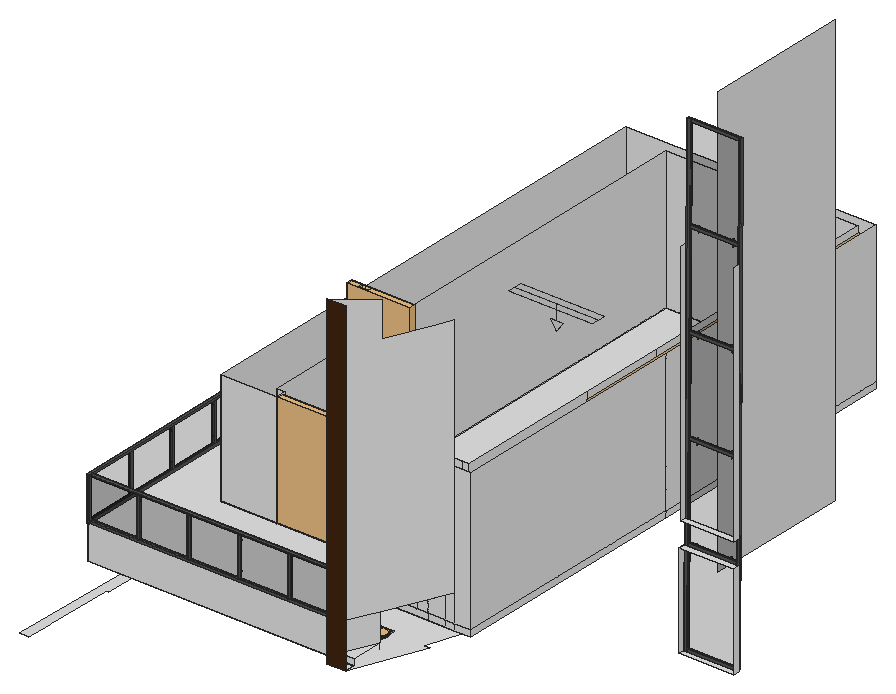
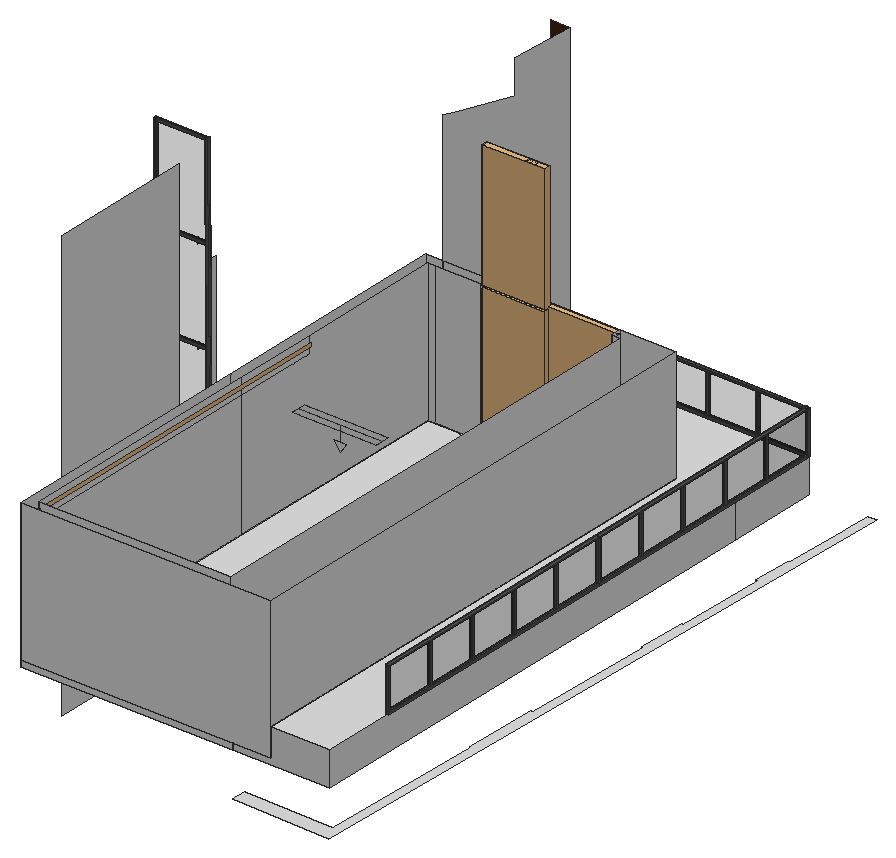
# SketchUp Ruby script. Lengths in inches.
U = 1.inch
M = Sketchup.active_model
def pt(a) = Geom::Point3d.new(a.map { |v| v * U })
def face(e, loops, mat)
  f = e.add_face(loops[0].map { |a| pt(a) })
  loops[1..].each { |l| e.add_face(l.map { |a| pt(a) }).erase! }
  f.material = f.back_material = mat if mat
  f
end
# faces: each face lists its corners as indices into pts; further lists are holes
def faces(e, pts, list, mat = nil) = list.each { |f| face(e, (f[0].is_a?(Array) ? f : [f]).map { |l| l.map { |i| pts[i] } }, mat) }
# xy, xz, yz: faces in a plane at the given z, y or x. An outline is a flat list of corners, or four numbers for a rectangle; further outlines are holes
def ring(l) = l.size == 4 ? [[l[0], l[1]], [l[2], l[1]], [l[2], l[3]], [l[0], l[3]]] : l.each_slice(2).to_a
def flat(e, list, mat, &to3) = list.each { |f| face(e, (f[0].is_a?(Array) ? f : [f]).map { |l| ring(l).map { |u, v| to3.(u, v) } }, mat) }
def xy(e, z, list, mat = nil) = flat(e, list, mat) { |x, y| [x, y, z] }
def xz(e, y, list, mat = nil) = flat(e, list, mat) { |x, z| [x, y, z] }
def yz(e, x, list, mat = nil) = flat(e, list, mat) { |y, z| [x, y, z] }
def lines(e, pts, list) = list.each { |a, b| e.add_line(pt(pts[a]), pt(pts[b])) }
# prism: a flat outline (further loops are holes) pulled along v
def prism(e, loops, v, mat = nil)
  f = face(e, loops, mat); d = Geom::Vector3d.new(v.map { |x| x * U })
  f.pushpull(f.normal.samedirection?(d) ? d.length : -d.length)
end
def box(e, o, s, mat = nil) = prism(e, [[o, [o[0] + s[0], o[1], o[2]], [o[0] + s[0], o[1] + s[1], o[2]], [o[0], o[1] + s[1], o[2]]]], [0, 0, s[2]], mat)
def at(x, y, z, deg = 0) = Geom::Transformation.translation(pt([x, y, z])) * Geom::Transformation.rotation(ORIGIN, Z_AXIS, deg.degrees)
def axes(o, x, y, z) = Geom::Transformation.new([*x, 0, *y, 0, *z, 0, *pt(o).to_a, 1])
def part(name) = M.definitions.add(name)
# library, detail: a bought-in or finely detailed component or shape, given as its bounding box
def library(name, o, s) = part(name).tap { |d| box(d.entities, o, s) }
def detail(e, o, s) = box(e.add_group.entities, o, s)
def put(e, d, t, mat = nil) = e.add_instance(d, t).tap { |i| i.material = mat if mat }
def group(e, t, mat = nil) = e.add_group.tap { |g| g.transformation = t; g.material = mat if mat }.entities
root = M.entities
M.materials.add("Aluminum_Polished").color = [83, 85, 85]
M.materials.add("Glass_Window_Neutral").color = [0, 0, 0]
M.materials["Glass_Window_Neutral"].alpha = 0.125
M.materials.add("Material~1").color = [0, 0, 0]
M.materials.add("[Color M03]").color = [226, 226, 226]
M.materials.add("[Color_001]").color = [196, 196, 196]
M.materials["[Color_001]"].alpha = 0.97
M.materials.add("[Wood Cherry Original]1").color = [66, 37, 18]
c1 = part("Group\#54")
box(c1.entities,[0,0,0],[2,1,28])
c2 = part("Group\#56")
p = [[0.11,0.32,0.14],[0.11,0.69,0.14]]
lines(c2.entities,p,[[0,1]])
g1 = group(c2.entities,at(0.11,0,0))
prism(g1,[[[0,0.24,0],[0,0.32,0.14],[0,0.24,0.27],[0,0.08,0.27],[0,0,0.14],[0,0.08,0]]],[-0.11,0,0])
c3 = part("Ver Glass Railing")
g2 = group(c3.entities,at(0,0,0),"Aluminum_Polished")
box(g2,[0,0,0],[2,185,2])
g3 = group(c3.entities,at(0,0,2),"Aluminum_Polished")
p = [[1.41,1,0],[1.41,36.8,0],[1.41,184,0],[1.29,184,0],[1.29,1,0],[1.29,36.8,0],
  [1.41,184,28],[1.29,184,28],[1.41,148.2,28],[1.29,148.2,28],[1.41,1,28],[1.29,1,28],
  [1.29,111.4,28],[1.29,111.4,0],[1.41,111.4,0],[1.41,111.4,28],[1.29,110.4,0],[1.29,110.4,28],
  [1.41,110.4,28],[1.41,110.4,0],[1.29,74.6,28],[1.29,74.6,0],[1.41,74.6,0],[1.41,74.6,28],
  [1.29,73.6,0],[1.29,73.6,28],[1.41,73.6,28],[1.41,73.6,0],[1.29,148.2,0],[1.41,148.2,0],
  [1.29,147.2,0],[1.29,147.2,28],[1.41,147.2,28],[1.41,147.2,0],[1.29,37.8,28],[1.29,37.8,0],
  [1.41,37.8,0],[1.41,37.8,28],[1.29,36.8,28],[1.41,36.8,28]]
lines(g3,p,[[0,1],[2,3],[4,5],[6,7],[6,8],[7,9],[10,11],[2,6],[3,7],[0,4],[11,4],[10,0],
  [12,13],[14,15],[16,17],[18,19],[20,21],[22,23],[24,25],[26,27],[27,22],[24,21],[23,26],[20,25],
  [9,28],[29,8],[30,31],[32,33],[33,29],[30,28],[8,32],[9,31],[34,35],[36,37],[5,38],[39,1],
  [1,36],[5,35],[37,39],[14,33],[19,14],[22,19],[36,27],[13,30],[16,13],[21,16],[35,24],[15,18],
  [12,17],[29,2],[28,3],[18,23],[32,15],[17,20],[31,12],[26,37],[25,34],[34,38],[39,10],[38,11]])
g4 = group(g3,at(1.79,1,0))
box(g4,[-0.5,0,0],[0.125,183,28],"Glass_Window_Neutral")
g5 = group(g3,at(0,184,28))
box(g5,[0,-184,0],[2.5,185,1])
put(g3,c1,axes([2,185,28],[-1,0,0],[0,-1,0],[0,0,-1]))
put(g3,c1,axes([2,1,28],[-1,0,0],[0,-1,0],[0,0,-1]))
put(g3,c1,axes([2,111.4,28],[-1,0,0],[0,-1,0],[0,0,-1]))
put(g3,c1,axes([2,74.6,28],[-1,0,0],[0,-1,0],[0,0,-1]))
g6 = group(g3,at(2,148.2,28))
box(g6,[-2,-1,-28],[2,1,28])
put(g3,c1,axes([2,37.8,28],[-1,0,0],[0,-1,0],[0,0,-1]))
put(g3,c2,at(1.17,146.31,24.26))
put(g3,c2,axes([1.17,148.89,24.54],[1,0,0],[0,-1,0],[0,0,-1]))
put(g3,c2,axes([1.17,148.89,4.79],[1,0,0],[0,-1,0],[0,0,-1]))
put(g3,c2,at(1.17,146.31,4.51))
put(g3,c2,at(1.17,109.51,4.51))
put(g3,c2,axes([1.17,112.09,4.79],[1,0,0],[0,-1,0],[0,0,-1]))
put(g3,c2,axes([1.17,112.09,24.54],[1,0,0],[0,-1,0],[0,0,-1]))
put(g3,c2,at(1.17,109.51,24.26))
put(g3,c2,axes([1.17,75.29,24.54],[1,0,0],[0,-1,0],[0,0,-1]))
put(g3,c2,at(1.17,72.71,4.51))
put(g3,c2,axes([1.17,75.29,4.79],[1,0,0],[0,-1,0],[0,0,-1]))
put(g3,c2,at(1.17,72.71,24.26))
put(g3,c2,axes([1.17,38.49,24.54],[1,0,0],[0,-1,0],[0,0,-1]))
put(g3,c2,at(1.17,35.91,4.51))
put(g3,c2,axes([1.17,38.49,4.79],[1,0,0],[0,-1,0],[0,0,-1]))
put(g3,c2,at(1.17,35.91,24.26))
c4 = part("Group259\#1")
p = [[0,0,0],[0,0,-6.22],[-2.62,0,-6.22],[17.05,-3.08,0],[-17.05,-3.08,0],[17.05,3.08,0],
  [17.05,0,0],[-17.05,3.08,0],[2.62,0,-6.22],[-17.05,0,0],[0,0,-10.0625]]
lines(c4.entities,p,[[0,1],[1,2],[3,4],[5,6],[7,5],[1,8],[9,0],[0,6],[8,10],[4,9],[6,3],[2,10],
  [9,7]])
c5 = part("Rectangle Light\#1")
put(c5.entities,c4,at(0,0,0))
c6 = library("Spot Light",[-5.1,-5.1,-11.05],[10.2,10.2,11.05])
c7 = library("Mesh Light\#8",[-0.5,-0.5,-0.1],[1,1,0.2])
c8 = library("Group\#3",[-0.5,-0.5,-0.1],[13,13,0.2])
c9 = library("Group11\#3",[-63.24,494.46,2.3125],[92.6,100.74,2109.15])
c10 = library("3DGeom~3_Defintion\#7",[-166.03,-457.45,-50.66],[409.15,1000,95.96])
c11 = part("Group12\#3")
put(c11.entities,c10,axes([-25.11,656.6,967.09],[0,1.68483,0],[0,0,2.10997],[-1.81292,0,0]),"Material~1")
c12 = part("Group10\#3")
put(c12.entities,c9,at(0,0,0),"[Color_001]")
put(c12.entities,c11,at(0,0,0))
c13 = library("Sliding Door",[0,0,0],[94.49,5.83,91.73])
c14 = library("Mesh Light\#7",[-0.5,-0.5,-0.1],[1,1,0.2])
xy(root,53.02,[[563.22,466.93,616.16,472.23]],"[Color M03]")
xy(root,123.23,[[244.05,83.53,244.68,107.8,243.62,107.83,245.35,174.72,247.41,174.67,248.39,212.13,246.32,212.18,248.6,299.78,250.22,299.74,251.43,346.17,249.8,346.21,253.15,475.08,254.77,475.04,256.62,546.02,254.99,546.0625,259.2,708.3,345.63,706.05,346,720.04,251.84,722.48,235.26,83.76]],"[Color M03]")
xy(root,144.21,[[563.22,466.93,616.16,472.23]],"[Color M03]")
xy(root,164.86,[[490.86,133.09,495.23,143.16,508.8,143.16,508.8,133.09]],"[Color M03]")
xy(root,165.42,[[[508.8,133.09,508.8,143.16,252.37,143.16,252.37,720.04,346,720.04,346,232.04,542.1,232.04,530.83,199.61,536.83,199.61],[495.02,187.63,496.58,187.84,498.02,188.4375,499.27,189.39,500.22,190.63,500.82,192.08,501.02,193.63,500.82,195.1875,500.22,196.63,499.27,197.875,498.02,198.83,496.58,199.43,495.02,199.63,493.47,199.43,492.02,198.83,490.78,197.875,489.83,196.63,489.23,195.1875,489.02,193.63,489.23,192.08,489.83,190.63,490.78,189.39,492.02,188.4375,493.47,187.84]],[346,232.04,356.8,232.04,356.8,242.01,355.97,242.01,355.97,710.07,540.52,710.07,540.52,242.01,510.66,242.01,533.7,232.04,550.5,232.04,550.5,720.04,346,720.04],[356.8,232.04,473.11,242.01],[473.11,232.04,498.76,232.04,503.08,242.01,473.11,242.01],[498.76,232.04,533.7,232.04,510.66,242.01,508.74,242.84,503.4375,242.84,503.08,242.01],
  [355.97,242.01,355.97,710.07,540.52,710.07,540.52,242.01,510.66,242.01,508.74,242.84,539.69,242.84,539.69,709.23,356.8,709.23,356.8,242.01],[356.8,242.01,473.11,242.84],[473.11,242.01,473.11,242.84,503.4375,242.84,503.08,242.01],[503.4375,242.84,504.27,244.78,508.74,242.84],[388.7,274.75,388.7,677.33,507.79,677.33,507.79,278.02,487.67,286.73,482.48,274.75]],"[Color M03]")
xy(root,167.67,[[564.58,466.93,616.16,472.23]],"[Color M03]")
xy(root,171.42,[[495.23,143.16,508.8,174.53,508.8,143.16],[309.43,232.04,346,720.04],[346,232.04,346,720.04,550.5,720.04,550.5,232.04,533.7,232.04,510.66,242.01,540.52,242.01,540.52,710.07,355.97,710.07,355.97,242.01,503.08,242.01,498.76,232.04],[498.76,232.04,533.7,232.04,510.66,242.01,503.08,242.01],[355.97,242.01,503.08,242.01,504.27,244.78,510.66,242.01,540.52,242.01,540.52,710.07,355.97,710.07],
  [503.08,242.01,510.66,242.01,504.27,244.78]],"[Color M03]")
xy(root,187.36,[[363.68,232.04,489.29,242.01]],"[Color M03]")
xy(root,198.23,[[252.37,143.16,495.23,143.16,508.8,174.53,533.7,232.04,309.43,232.04,309.43,720.04,252.37,720.04]],"[Color M03]")
xz(root,133.09,[[490.86,164.86,508.8,479.92]],"[Wood Cherry Original]1")
xz(root,143.16,[[495.23,164.86,508.8,165.42],[252.37,165.42,495.23,198.23],[495.23,165.42,508.8,171.42]],"[Color M03]")
xz(root,232.04,[[346,165.42,508.8,171.42],[508.8,165.42,525.57,171.42],[525.57,165.42,533.7,171.42],[533.7,165.42,550.5,171.42],[309.43,171.42,346,198.23],
  [346,171.42,498.76,171.42,498.76,198.23,489.29,198.23,489.29,187.36,363.68,187.36,363.68,198.23,346,198.23],[498.76,171.42,508.8,198.23],[508.8,171.42,525.57,198.23],[525.57,171.42,533.7,198.23],[533.7,171.42,550.5,306.98],
  [363.68,187.36,489.29,198.23],[309.43,198.23,363.68,306.98],[489.29,198.23,533.7,306.98]],"[Color M03]")
xz(root,242.01,[[355.97,165.42,503.08,171.42],[510.66,165.42,533.7,171.42],[533.7,165.42,540.52,171.42],[355.97,171.42,355.97,306.98,363.68,306.98,363.68,187.36,489.29,187.36,489.29,306.98,533.7,306.98,533.7,171.42],[533.7,171.42,540.52,306.98]],"[Color M03]")
xz(root,710.07,[[355.97,165.42,540.52,171.42],[355.97,171.42,540.52,306.98]],"[Color M03]")
xz(root,720.04,[[252.37,165.42,252.37,198.23,309.43,198.23,309.43,171.42,346,171.42,346,165.42],[346,165.42,550.5,171.42],[309.43,171.42,550.5,306.98]],"[Color M03]")
yz(root,252.37,[[143.16,165.42,232.04,198.23],[232.04,165.42,720.04,198.23]],"[Color M03]")
yz(root,309.43,[[232.04,171.42,720.04,198.23],[232.04,198.23,720.04,306.98]],"[Color M03]")
yz(root,346,[[232.04,165.42,720.04,171.42]],"[Color M03]")
yz(root,355.97,[[242.01,165.42,710.07,171.42],[242.01,171.42,710.07,306.98]],"[Color M03]")
yz(root,363.68,[[232.04,187.36,242.01,306.98]],"[Color M03]")
yz(root,489.29,[[232.04,187.36,242.01,306.98]],"[Color M03]")
yz(root,508.8,[[133.09,164.86,143.16,165.42]],"[Color M03]")
yz(root,540.52,[[242.01,165.42,466.93,171.42],[466.93,165.42,710.07,171.42],[242.01,171.42,242.01,306.98,383.94,306.98,383.94,291.23,466.93,291.23,466.93,171.42],[466.93,171.42,710.07,291.23]],"[Color M03]")
yz(root,550.5,[[232.04,165.42,466.93,171.42],[466.93,165.42,720.04,171.42],[232.04,171.42,466.93,306.98],[466.93,171.42,720.04,306.98]],"[Color M03]")
yz(root,555.8,[[522.82,96,663.25,510.46]],"[Color M03]")
yz(root,563.22,[[466.93,53.02,472.23,144.21]],"[Color M03]")
yz(root,564.58,[[466.93,167.67,472.23,404.08]],"[Color M03]")
yz(root,616.16,[[466.93,53.02,472.23,144.21],[466.93,167.67,472.23,404.08]],"[Color M03]")
p = [[490.86,133.09,164.86],[490.86,133.09,479.92],[509.46,176.05,466.59],[509.46,176.05,432.98],[528.06,219.01,432.98],[533.7,232.04,432.98],
  [533.7,232.04,328.48],[533.7,232.04,312.98],[533.7,232.04,306.98],[533.7,232.04,198.23],[508.8,174.53,198.23],[495.23,143.16,198.23],
  [495.23,143.16,171.42],[495.23,143.16,165.42],[495.23,143.16,164.86],[495.02,187.63,165.42],[493.47,187.84,165.42],[493.47,187.84,167.29],
  [495.02,187.63,167.29],[496.58,187.84,165.42],[496.58,187.84,167.29],[492.02,188.4375,165.42],[492.02,188.4375,167.29],[498.02,188.4375,165.42],
  [498.02,188.4375,167.29],[490.78,189.39,165.42],[490.78,189.39,167.29],[499.27,189.39,165.42],[499.27,189.39,167.29],[489.83,190.63,165.42],
  [489.83,190.63,167.29],[500.22,190.63,165.42],[500.22,190.63,167.29],[489.23,192.08,165.42],[489.23,192.08,167.29],[500.82,192.08,165.42],
  [500.82,192.08,167.29],[489.02,193.63,165.42],[489.02,193.63,167.29],[501.02,193.63,165.42],[501.02,193.63,167.29],[489.23,195.1875,165.42],
  [489.23,195.1875,167.29],[500.82,195.1875,165.42],[500.82,195.1875,167.29],[489.83,196.63,165.42],[489.83,196.63,167.29],[500.22,196.63,165.42],
  [500.22,196.63,167.29],[490.78,197.875,165.42],[490.78,197.875,167.29],[499.27,197.875,165.42],[499.27,197.875,167.29],[492.02,198.83,165.42],
  [492.02,198.83,167.29],[498.02,198.83,165.42],[498.02,198.83,167.29],[493.47,199.43,165.42],[493.47,199.43,167.29],[496.58,199.43,165.42],
  [496.58,199.43,167.29],[495.02,199.63,165.42],[495.02,199.63,167.29],[533.7,232.04,165.42],[510.66,242.01,165.42],[510.66,242.01,171.42],
  [533.7,232.04,171.42],[503.08,242.01,171.42],[503.08,242.01,165.42],[503.4375,242.84,165.42],[504.27,244.78,165.42],[504.27,244.78,171.42],
  [508.74,242.84,165.42],[508.8,174.53,171.42],[508.8,174.53,165.42],[479.38,187.26,171.42],[479.38,187.26,165.42],[356.8,232.04,165.42],
  [356.8,232.49,160.38],[473.11,232.49,160.38],[473.11,232.04,165.42]]
faces(root,p,[[0,1,2,3,4,5,6,7,8,9,10,11,12,13,14],[15,16,17,18],[19,15,18,20],[16,21,22,17],[23,19,20,24],[21,25,26,22],[27,23,24,28],[25,29,30,26],
  [31,27,28,32],[29,33,34,30],[35,31,32,36],[33,37,38,34],[39,35,36,40],[37,41,42,38],[43,39,40,44],[41,45,46,42],
  [47,43,44,48],[45,49,50,46],[51,47,48,52],[49,53,54,50],[55,51,52,56],[53,57,58,54],[59,55,56,60],[57,61,62,58],
  [61,59,60,62],[63,64,65,66],[67,68,69,70,71],[71,65,64,72,70],[73,12,11,10]],"[Color M03]")
lines(root,p,[[73,74],[75,76],[77,78],[79,80]])
put(root,c3,axes([563.22,472.23,53.02],[0,0.99996,-0.00929],[0,0.02298,2.47401],[1.66784,0,0]),"[Color M03]")
put(root,c5,axes([444.17,483.33,164.92],[2.37,0,0],[0,2.37,0],[0,0,2.37]))
put(root,c6,at(495.02,193.63,166.78),"[Color M03]")
g7 = group(root,at(356.8,242.84,165.42))
xy(g7,0,[[[0,0,0,466.39,182.89,466.39,182.89,0,151.94,0,147.47,1.93,146.64,0],[31.9,31.9,125.68,31.9,130.87,43.89,150.99,35.18,150.99,434.49,31.9,434.49]]],"[Color M03]")
put(g7,c7,axes([91.45,233.2,0],[183.89359,0,0],[0,467.39359,0],[0,0,1]))
put(root,c8,at(489.02,187.63,167.29),"[Color M03]")
put(root,c12,axes([395.51,238.49,183.26],[0,0.03519,0],[0.08781,0,0],[0,0,0.05732]),"[Color_001]")
put(root,c13,axes([363.68,232.04,187.36],[1.32932,0,0],[0,1,0],[0,0,1.30407]),"[Color M03]")
put(root,c3,axes([495.23,143.16,198.23],[0,1.37,0],[-1.31773,0,0],[0,0,1.37]),"[Color M03]")
put(root,c3,axes([251.45,143.16,198.23],[1.37,0,0],[0,1.37,0],[0,0,1.37]),"[Color M03]")
put(root,c3,axes([251.45,396.61,198.23],[1.37,0,0],[0,1.37,0],[0,0,1.37]),"[Color M03]")
put(root,c5,axes([437.61,476.14,306.48],[2.37,0,0],[0,2.37,0],[0,0,2.37]))
g8 = group(root,at(540.52,383.94,291.23))
yz(g8,0,[[0,0,82.99,15.75],[82.99,0,326.125,15.75]],"[Color M03]")
put(g8,c14,axes([0,163.0625,7.875],[1,0,0],[0,327.125,0],[0,0,16.75]))
put(root,c12,axes([395.51,238.49,305.79],[0,0.03519,0],[0.08781,0,0],[0,0,0.05732]),"[Color_001]")
